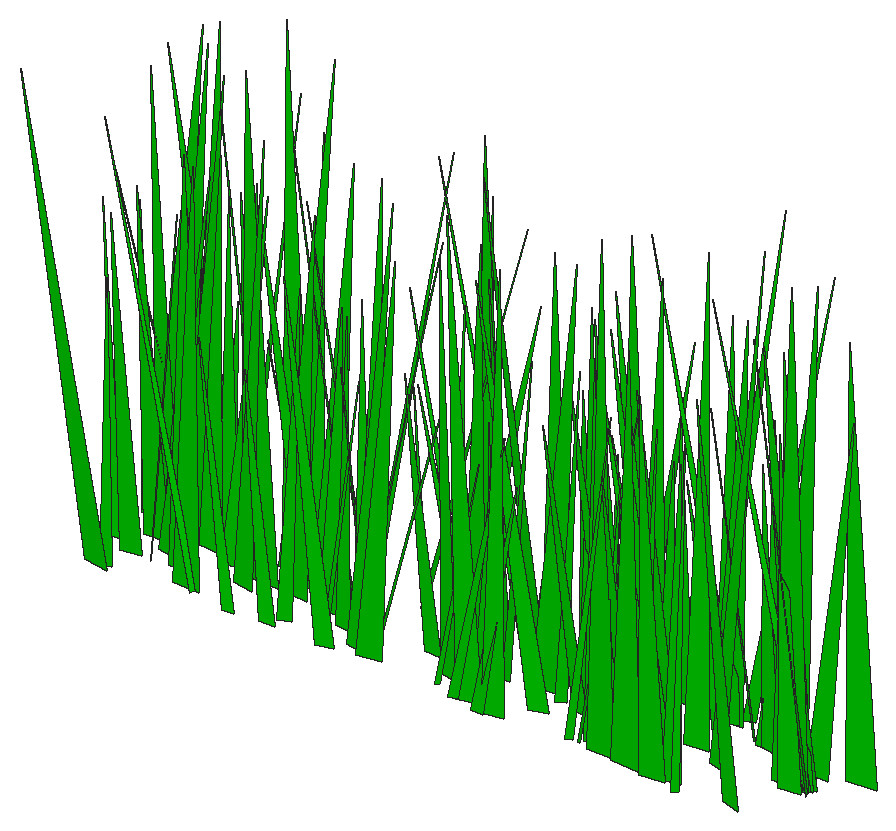
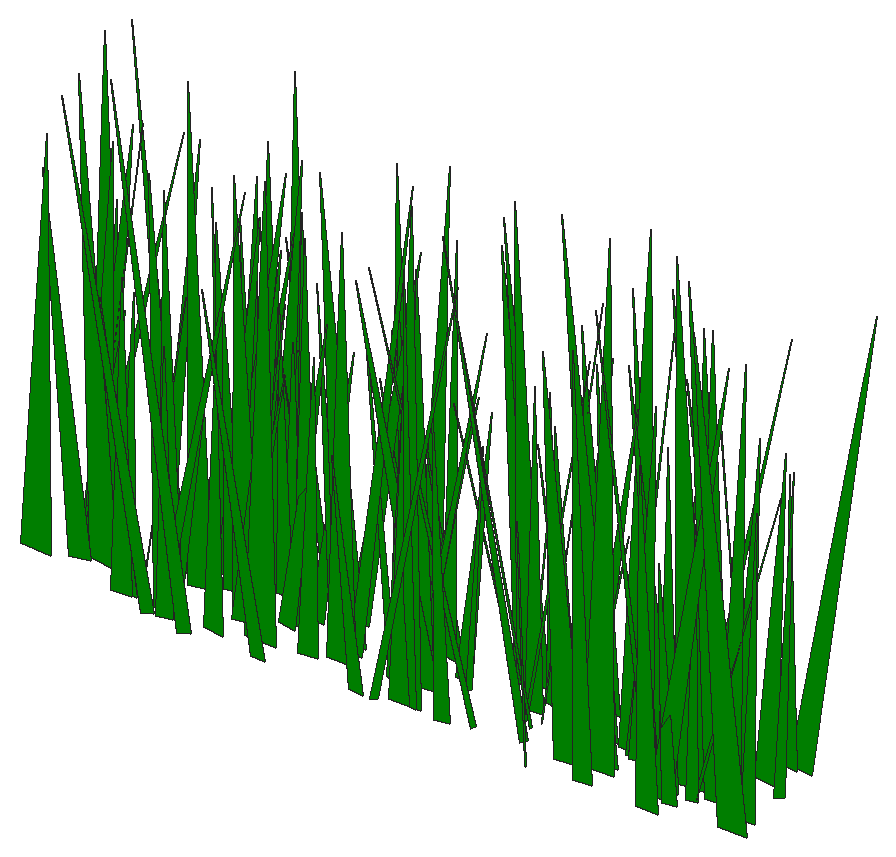
# SketchUp Ruby script. Lengths in inches.
U = 1.inch
M = Sketchup.active_model
def pt(a) = Geom::Point3d.new(a.map { |v| v * U })
def face(e, loops, mat)
  f = e.add_face(loops[0].map { |a| pt(a) })
  loops[1..].each { |l| e.add_face(l.map { |a| pt(a) }).erase! }
  f.material = f.back_material = mat if mat
  f
end
# faces: each face lists its corners as indices into pts; further lists are holes
def faces(e, pts, list, mat = nil) = list.each { |f| face(e, (f[0].is_a?(Array) ? f : [f]).map { |l| l.map { |i| pts[i] } }, mat) }
# xy, xz, yz: faces in a plane at the given z, y or x. An outline is a flat list of corners, or four numbers for a rectangle; further outlines are holes
def ring(l) = l.size == 4 ? [[l[0], l[1]], [l[2], l[1]], [l[2], l[3]], [l[0], l[3]]] : l.each_slice(2).to_a
def flat(e, list, mat, &to3) = list.each { |f| face(e, (f[0].is_a?(Array) ? f : [f]).map { |l| ring(l).map { |u, v| to3.(u, v) } }, mat) }
def xy(e, z, list, mat = nil) = flat(e, list, mat) { |x, y| [x, y, z] }
def xz(e, y, list, mat = nil) = flat(e, list, mat) { |x, z| [x, y, z] }
def yz(e, x, list, mat = nil) = flat(e, list, mat) { |y, z| [x, y, z] }
def lines(e, pts, list) = list.each { |a, b| e.add_line(pt(pts[a]), pt(pts[b])) }
# prism: a flat outline (further loops are holes) pulled along v
def prism(e, loops, v, mat = nil)
  f = face(e, loops, mat); d = Geom::Vector3d.new(v.map { |x| x * U })
  f.pushpull(f.normal.samedirection?(d) ? d.length : -d.length)
end
def box(e, o, s, mat = nil) = prism(e, [[o, [o[0] + s[0], o[1], o[2]], [o[0] + s[0], o[1] + s[1], o[2]], [o[0], o[1] + s[1], o[2]]]], [0, 0, s[2]], mat)
def at(x, y, z, deg = 0) = Geom::Transformation.translation(pt([x, y, z])) * Geom::Transformation.rotation(ORIGIN, Z_AXIS, deg.degrees)
def axes(o, x, y, z) = Geom::Transformation.new([*x, 0, *y, 0, *z, 0, *pt(o).to_a, 1])
def part(name) = M.definitions.add(name)
# library, detail: a bought-in or finely detailed component or shape, given as its bounding box
def library(name, o, s) = part(name).tap { |d| box(d.entities, o, s) }
def detail(e, o, s) = box(e.add_group.entities, o, s)
def put(e, d, t, mat = nil) = e.add_instance(d, t).tap { |i| i.material = mat if mat }
def group(e, t, mat = nil) = e.add_group.tap { |g| g.transformation = t; g.material = mat if mat }.entities
root = M.entities
M.materials.add("[Color G06]").color = [0, 204, 0]
c1 = part("fur_instance\#9")
p = [[0.8125,0,1.79],[0.67,-0.02,1.48],[0,-0.11,0],[0,0.11,0]]
faces(c1.entities,p,[[0,1,2,3]])
put(root,c1,axes([12.97,15.97,4.28],[-3.99337,-0.56787,0.77876],[-4.0854,0.55967,0.08592],[0.40602,0.04624,8.52399]),"[Color G06]")
put(root,c1,axes([12.24,19.35,4.28],[-2.73791,0.24663,2.09563],[1.98216,0.40975,0.245],[1.07946,-0.12686,4.86539]),"[Color G06]")
put(root,c1,axes([12.44,17.64,4.28],[-3.32975,0.20415,1.76228],[1.47677,0.49102,-0.30149],[1.16308,-0.03901,5.42796]),"[Color G06]")
put(root,c1,axes([14.24,19.35,4.28],[-4.0614,-0.11884,0.09777],[-0.84903,0.56603,0.25097],[0.09846,-0.02105,6.19718]),"[Color G06]")
put(root,c1,axes([12.99,19.34,4.28],[-2.92814,-0.56418,2.22224],[-4.18418,0.43225,0.29114],[1.03573,0.15122,7.45871]),"[Color G06]")
put(root,c1,axes([12.22,20.1,4.28],[2.30465,0.69491,2.08222],[5.1631,-0.32291,-0.38533],[-0.34273,-0.1917,8.19688]),"[Color G06]")
put(root,c1,axes([13.31,17.18,4.28],[-0.75917,-0.50042,1.73825],[-3.77236,0.09965,-0.38475],[-0.0241,0.16607,5.46872]),"[Color G06]")
put(root,c1,axes([13.37,18.3125,4.28],[-0.04547,-0.61844,0.06629],[-4.4314,0.00608,-0.27434],[-0.1831,0.00644,6.62305]),"[Color G06]")
put(root,c1,axes([13.24,16.09,4.28],[2.66433,-0.22899,1.74164],[-1.66367,-0.40217,-0.38923],[-1.13439,0.05198,4.66142]),"[Color G06]")
put(root,c1,axes([15.12,19.87,4.28],[-4.34443,0.46349,1.04288],[3.36999,0.60791,0.32271],[0.4215,-0.08318,8.16905]),"[Color G06]")
put(root,c1,axes([14.3,19.41,4.28],[-2.26458,0.22299,1.73631],[1.73449,0.34233,0.00285],[0.9478,-0.09368,4.14335]),"[Color G06]")
put(root,c1,axes([13.57,19.03,4.28],[3.79606,-0.59816,1.93914],[-4.37494,-0.54602,-0.21773],[-0.97142,0.12164,8.55822]),"[Color G06]")
put(root,c1,axes([16.17,16.53,4.28],[-5.20829,0.09415,0.81442],[0.69711,0.72939,0.2722],[0.51653,-0.03508,7.84458]),"[Color G06]")
put(root,c1,axes([14.06,17.17,4.28],[3.87029,0.05666,1.82111],[0.36921,-0.56575,0.26912],[-1.23022,0.00845,5.80998]),"[Color G06]")
put(root,c1,axes([14.07,17.84,4.28],[3.71321,0.3398,1.42529],[2.48378,-0.53033,0.06985],[-0.82348,-0.06738,6.63758]),"[Color G06]")
put(root,c1,axes([14.67,19.98,4.28],[1.18507,-0.32203,1.12325],[-2.4133,-0.16921,0.11452],[-0.27201,0.09828,3.87775]),"[Color G06]")
put(root,c1,axes([14.76,18.81,4.28],[-0.00288,0.78852,3.16986],[6.0329,0.01406,-0.38965],[0.27952,-0.29542,8.4424]),"[Color G06]")
put(root,c1,axes([14.98,20.64,4.28],[-0.50165,-0.47813,2.71106],[-3.86307,0.08472,0.1197],[0.35197,0.24839,5.1778]),"[Color G06]")
put(root,c1,axes([14.48,18.375,4.28],[3.8157,0.52747,2.29269],[3.94724,-0.5514,-0.10152],[-1.0396,-0.15758,8.02953]),"[Color G06]")
put(root,c1,axes([15.18,19.41,4.28],[2.12266,-0.39029,2.66699],[-3.16809,-0.32635,0.14609],[-0.99052,0.20743,5.24802]),"[Color G06]")
put(root,c1,axes([15.22,17.28,4.28],[0.01322,-0.6977,1.04536],[-5.04951,0.00129,0.24114],[0.16106,0.09754,7.47412]),"[Color G06]")
put(root,c1,axes([15.85,16.57,4.28],[1.1157,0.61922,2.23173],[4.66513,-0.1665,0.09743],[-0.43033,-0.1996,6.84238]),"[Color G06]")
put(root,c1,axes([15.36,20.01,4.28],[5.25298,-0.04802,1.83643],[-0.34875,-0.75223,-0.03124],[-1.22749,0.00822,7.86775]),"[Color G06]")
put(root,c1,axes([16.93,18.49,4.28],[-1.99698,0.53565,0.90443],[3.86216,0.28426,-0.29118],[0.45339,-0.06214,6.46403]),"[Color G06]")
put(root,c1,axes([17.51,18.43,4.28],[-5.08262,-0.02922,1.9462],[-0.14859,0.73101,0.39401],[1.31053,-0.03044,7.59258]),"[Color G06]")
put(root,c1,axes([16.02,18.39,4.28],[3.71946,-0.31875,1.53864],[-2.36483,-0.53136,0.12424],[-0.83221,0.0853,6.52372]),"[Color G06]")
put(root,c1,axes([17.72,16.2,4.28],[-2.50517,0.23981,0.70508],[1.72266,0.35476,-0.18919],[0.4611,-0.02247,4.53757]),"[Color G06]")
put(root,c1,axes([17.32,18.19,4.28],[-0.30423,-0.86212,0.93414],[-6.21332,0.04351,0.09236],[0.09275,0.08662,9.25092]),"[Color G06]")
put(root,c1,axes([17.55,19.71,4.28],[-3.56106,0.6221,3.38706],[4.81861,0.53089,0.11525],[1.34882,-0.25418,8.53056]),"[Color G06]")
put(root,c1,axes([17.12,17.66,4.28],[3.69725,0.44313,2.60223],[3.39482,-0.54489,-0.11494],[-1.26701,-0.16687,7.28555]),"[Color G06]")
put(root,c1,axes([18.66,18.76,4.28],[-3.42525,0.34148,0.96228],[2.48879,0.48185,0.14553],[0.46633,-0.06338,6.29139]),"[Color G06]")
put(root,c1,axes([17.48,20.53,4.28],[-3.57875,0.32608,3.47096],[2.71455,0.56274,0.1788],[1.86891,-0.19296,6.38681]),"[Color G06]")
put(root,c1,axes([18.64,18.99,4.28],[-2.60474,-0.11719,0.41893],[-0.83062,0.36527,0.2014],[0.30803,-0.00599,4.08561]),"[Color G06]")
put(root,c1,axes([17.59,19.36,4.28],[-3.88057,0.44362,5.32366],[3.90711,0.66294,0.01572],[2.74645,-0.31629,7.49964]),"[Color G06]")
put(root,c1,axes([19.05,16.35,4.28],[-1.44782,0.36298,0.04776],[2.60234,0.20194,-0.088],[0.06699,0.0001,4.45081]),"[Color G06]")
put(root,c1,axes([18.53,19.875,4.28],[0.32232,0.67897,0.85695],[4.8979,-0.04104,-0.3795],[0.21728,-0.08203,7.28323]),"[Color G06]")
put(root,c1,axes([18.58,18.17,4.28],[1.04511,-0.6508,0.62458],[-4.68306,-0.14307,0.37927],[0.15738,0.06455,7.13791]),"[Color G06]")
put(root,c1,axes([20.64,18.48,4.28],[-5.04728,-0.06519,1.53889],[-0.4679,0.71828,0.06742],[1.02946,0.00685,7.57553]),"[Color G06]")
put(root,c1,axes([19.39,20.82,4.28],[2.51743,0.06611,1.50259],[0.57866,-0.37429,-0.27395],[-0.94903,-0.05286,3.8188]),"[Color G06]")
put(root,c1,axes([19.35,16.8125,4.28],[3.03443,-0.31056,1.66408],[-2.27883,-0.44502,-0.25852],[-1.00338,0.07149,5.61967]),"[Color G06]")
put(root,c1,axes([21.03,18.76,4.28],[-4.51249,0.00468,1.04323],[0.02243,0.63665,-0.11127],[0.69846,0.00978,6.74352]),"[Color G06]")
put(root,c1,axes([20.08,18.02,4.28],[0.23374,0.52169,0.02925],[3.74089,-0.03263,0.07414],[-0.05073,-0.00229,5.60188]),"[Color G06]")
put(root,c1,axes([21.22,16.33,4.28],[-2.97507,0.39241,0.93894],[2.85386,0.41871,0.09665],[0.41139,-0.06682,6.11972]),"[Color G06]")
put(root,c1,axes([20.39,17.47,4.28],[2.87267,-0.04954,0.94055],[-0.36714,-0.40987,0.02501],[-0.62244,0.01314,4.32605]),"[Color G06]")
put(root,c1,axes([20.95,17.52,4.28],[2.15661,0.34791,2.0146],[2.6896,-0.32579,0.03183],[-0.89886,-0.1401,4.9288]),"[Color G06]")
put(root,c1,axes([21.24,18.13,4.28],[-2.20847,0.34506,2.4406],[2.79412,0.33718,0.17148],[0.99128,-0.18166,4.95408]),"[Color G06]")
put(root,c1,axes([21.89,17.42,4.28],[-2.90538,-0.03584,1.2201],[-0.2819,0.42045,-0.08058],[0.80811,0.01781,4.35853]),"[Color G06]")
put(root,c1,axes([20.33,19.71,4.28],[5.4871,-0.11222,1.2148],[-0.82981,-0.77282,0.17144],[-0.78721,0.03244,8.28684]),"[Color G06]")
put(root,c1,axes([20.67,18.96,4.28],[4.7064,0.0037,0.7795],[0.04286,-0.65997,-0.21778],[-0.52047,-0.02085,7.03079]),"[Color G06]")
put(root,c1,axes([22.3125,16.98,4.28],[-3.43987,0.47523,3.74009],[3.79084,0.54588,-0.17991],[1.87253,-0.2321,7.23484]),"[Color G06]")
put(root,c1,axes([22.05,16.8,4.28],[3.64569,0.49267,2.10372],[3.67873,-0.52579,-0.09533],[-0.96466,-0.14321,7.58698]),"[Color G06]")
put(root,c1,axes([22.95,20.28,4.28],[2.39811,-0.32059,1.90981],[-2.47886,-0.3561,0.08587],[-0.87967,0.12949,4.96445]),"[Color G06]")
put(root,c1,axes([23.5,18.3125,4.28],[-2.61944,0.11067,1.29609],[0.79209,0.3844,-0.19463],[0.86861,-0.01679,4.08605]),"[Color G06]")
put(root,c1,axes([22.67,16.6,4.28],[2.58776,-0.57387,1.0544],[-4.14768,-0.36661,-0.18318],[-0.48026,0.07406,7.26333]),"[Color G06]")
put(root,c1,axes([23.98,17.95,4.28],[-1.29592,-0.41524,0.6149],[-3.0044,0.181,-0.1027],[0.10063,0.05645,4.85264]),"[Color G06]")
put(root,c1,axes([22.4,17.375,4.28],[3.16952,0.08118,0.18889],[0.58245,-0.44232,0.00692],[-0.12514,-0.00255,4.81633]),"[Color G06]")
put(root,c1,axes([25.35,20.44,4.28],[-5.24058,0.10532,0.92421],[0.76645,0.73558,0.0781],[0.60452,-0.01956,7.91298]),"[Color G06]")
put(root,c1,axes([22,19.98,4.28],[5.15965,-0.04603,0.24118],[-0.3322,-0.71977,0.09534],[-0.15695,0.01032,7.72665]),"[Color G06]")
put(root,c1,axes([25.55,17.91,4.28],[-4.16168,0.10609,0.76813],[0.76342,0.58466,-0.03662],[0.50999,-0.0095,6.3229]),"[Color G06]")
put(root,c1,axes([24.23,20.17,4.28],[3.89408,0.32417,2.95544],[2.58214,-0.58824,-0.1877],[-1.62702,-0.1577,6.77562]),"[Color G06]")
put(root,c1,axes([24.41,20.16,4.28],[-1.14896,-0.74215,2.53014],[-5.56478,0.17257,0.17026],[0.47377,0.22719,8.13583]),"[Color G06]")
put(root,c1,axes([24.89,18.74,4.28],[2.16476,0.52445,2.62984],[4.06025,-0.32528,-0.01402],[-0.86901,-0.21336,6.48561]),"[Color G06]")
put(root,c1,axes([26.1,17.25,4.28],[-2.88067,0.24068,0.35111],[1.7402,0.40043,0.36019],[0.07683,-0.04569,5.00608]),"[Color G06]")
put(root,c1,axes([25.18,17.17,4.28],[3.36748,0.36101,3.26227],[2.94574,-0.52402,-0.13064],[-1.67019,-0.19634,6.34706]),"[Color G06]")
put(root,c1,axes([25.68,19.23,4.28],[-3.57116,-0.23033,2.25433],[-1.85175,0.52669,-0.37073],[1.25476,0.12174,5.86893]),"[Color G06]")
put(root,c1,axes([24.4,19.02,4.28],[3.76842,-0.38067,0.08752],[-2.7303,-0.52551,0.02879],[-0.03612,0.00697,6.95467]),"[Color G06]")
put(root,c1,axes([26.02,18.2,4.28],[-2.36297,-0.15451,1.64195],[-1.20853,0.35708,-0.02501],[0.98696,0.06733,3.90053]),"[Color G06]")
put(root,c1,axes([25.16,16.67,4.28],[2.75052,-0.07469,0.51501],[-0.53119,-0.38654,-0.10239],[-0.35132,-0.00027,4.18681]),"[Color G06]")
put(root,c1,axes([26.57,16.4,4.28],[-3.66563,0.4997,2.75267],[3.85257,0.53635,0.27512],[1.17942,-0.19892,7.65655]),"[Color G06]")
put(root,c1,axes([26,20.48,4.28],[1.29119,0.3455,0.36803],[2.48288,-0.18156,0.12241],[-0.18666,-0.02514,4.17395]),"[Color G06]")
put(root,c1,axes([27.44,18.71,4.28],[-4.81347,-0.39314,1.65522],[-2.82911,0.6871,0.36968],[1.08214,0.04763,8.32904]),"[Color G06]")
put(root,c1,axes([26.52,17.24,4.28],[1.15356,-0.50879,1.09317],[-3.71894,-0.16141,0.13585],[-0.13219,0.10111,5.71768]),"[Color G06]")
put(root,c1,axes([26.58,18.1,4.28],[3.17916,0.25116,1.41806],[1.79703,-0.46151,0.39087],[-0.9566,-0.03227,5.44706]),"[Color G06]")
put(root,c1,axes([26.05,16.3,4.28],[3.09991,-0.2022,0.39382],[-1.45116,-0.43371,-0.06535],[-0.25724,0.01003,5.11445]),"[Color G06]")
put(root,c1,axes([28.51,17.21,4.28],[-3.71731,0.43062,0.59629],[3.10304,0.5195,0.11403],[0.25793,-0.04376,7.22186]),"[Color G06]")
put(root,c1,axes([27.46,19.34,4.28],[0.04217,-0.66337,1.82671],[-4.91117,-0.00322,0.11907],[0.07142,0.17051,7.10924]),"[Color G06]")
put(root,c1,axes([27.13,16.07,4.28],[1.7386,0.32911,0.00623],[2.35863,-0.24231,0.15265],[-0.0847,0.00798,4.37852]),"[Color G06]")
put(root,c1,axes([27.62,16.17,4.28],[3.51083,-0.45343,2.81826],[-3.48747,-0.52717,-0.03872],[-1.40235,0.17582,7.15191]),"[Color G06]")
put(root,c1,axes([28.45,19.65,4.28],[-0.43724,-0.48819,0.48954],[-3.50938,0.06346,0.26863],[0.21966,0.04214,5.26624]),"[Color G06]")
put(root,c1,axes([27.9,18.34,4.28],[2.19793,-0.70483,0.35704],[-5.05855,-0.30697,-0.05166],[-0.12699,0.02862,8.23749]),"[Color G06]")
put(root,c1,axes([29.52,17.89,4.28],[-1.98109,-0.37435,0.48553],[-2.69363,0.27813,0.08393],[0.23827,0.03177,4.9858]),"[Color G06]")
put(root,c1,axes([28.68,18.0625,4.28],[3.38444,-0.21962,1.72049],[-1.60433,-0.49622,-0.22711],[-1.10991,0.04757,5.57456]),"[Color G06]")
put(root,c1,axes([30.04,18.66,4.28],[-2.17423,-0.41258,0.76693],[-2.99199,0.30516,-0.08877],[0.2555,0.06261,5.48688]),"[Color G06]")
put(root,c1,axes([29.46,18.51,4.28],[1.2325,0.57157,2.16422],[4.30418,-0.18989,0.28582],[-0.60989,-0.18507,6.39069]),"[Color G06]")
put(root,c1,axes([30.09,19.84,4.28],[-0.15315,-0.68705,2.67581],[-5.24219,0.0209,-0.05361],[0.01748,0.24969,7.36715]),"[Color G06]")
put(root,c1,axes([31.13,19.22,4.28],[-2.47487,0.59914,0.02513],[4.29363,0.34497,-0.26384],[0.16136,0.01026,7.40604]),"[Color G06]")
put(root,c1,axes([29.47,20.71,4.28],[3.1825,0.36757,0.87629],[2.67812,-0.44581,-0.24469],[-0.34571,-0.06987,6.17127]),"[Color G06]")
put(root,c1,axes([31.43,19.1,4.28],[-2.67538,0.22308,0.53204],[1.62152,0.3741,0.19492],[0.23789,-0.04116,4.65479]),"[Color G06]")
put(root,c1,axes([30.94,16.72,4.28],[3.06671,-0.33736,2.7629],[-2.72528,-0.46729,0.20242],[-1.35768,0.17597,5.83448]),"[Color G06]")
put(root,c1,axes([30.23,16.48,4.28],[3.76639,-0.13217,1.20525],[-0.96093,-0.53663,-0.05273],[-0.79079,0.02257,5.80443]),"[Color G06]")
put(root,c1,axes([31.22,17.27,4.28],[1.97021,-0.33519,1.64699],[-2.53812,-0.29348,-0.07908],[-0.74188,0.11387,4.64449]),"[Color G06]")
put(root,c1,axes([31.5,16.57,4.28],[-0.15398,0.42548,0.18327],[3.05228,0.02093,0.1467],[-0.09193,-0.01776,4.56368]),"[Color G06]")
put(root,c1,axes([31.52,20.23,4.28],[0.65567,0.43101,1.35597],[3.19532,-0.10338,0.32354],[-0.40815,-0.11695,4.71125]),"[Color G06]")
put(root,c1,axes([31.47,16.4,4.28],[3.0712,0.62728,3.17092],[4.76894,-0.47012,0.36582],[-1.41202,-0.22343,8.13241]),"[Color G06]")
put(root,c1,axes([31.38,18.82,4.28],[1.0346,0.69031,1.49059],[5.03848,-0.15064,0.20224],[-0.33896,-0.13215,7.5559]),"[Color G06]")
put(root,c1,axes([31.55,17.25,4.28],[0.61246,-0.35566,1.05629],[-2.63957,-0.08948,-0.04241],[-0.19359,0.09487,3.92012]),"[Color G06]")
put(root,c1,axes([32.17,16.46,4.28],[2.68438,-0.43992,3.9778],[-3.71413,-0.45057,-0.12542],[-1.80038,0.27358,6.18967]),"[Color G06]")
put(root,c1,axes([30.58,16.52,4.28],[4.05523,0.12048,0.92255],[0.841,-0.57188,0.32168],[-0.64825,0.01177,6.18851]),"[Color G06]")
put(root,c1,axes([32.29,17.36,4.28],[-3.02264,-0.17933,1.20075],[-1.30641,0.43482,0.11388],[0.76979,0.03378,4.90811]),"[Color G06]")
put(root,c1,axes([31.48,16.47,4.28],[2.58244,-0.19784,1.46172],[-1.53046,-0.37624,0.18993],[-0.7919,0.08197,4.39967]),"[Color G06]")
put(root,c1,axes([33.46,20.23,4.28],[-5.24909,0.19126,0.84342],[1.36531,0.73618,-0.1972],[0.57936,-0.00199,8.10616]),"[Color G06]")
put(root,c1,axes([32.34,16.59,4.28],[-1.46668,-0.43821,0.1902],[-3.13231,0.20529,0.37872],[0.28345,0.00108,5.16925]),"[Color G06]")
put(root,c1,axes([33.47,16.6,4.28],[-3.5207,0.32723,0.7119],[2.36649,0.49352,0.08366],[0.36508,-0.04337,6.32309]),"[Color G06]")
put(root,c1,axes([33.58,16.64,4.28],[-3.31135,0.51856,0.73563],[3.73861,0.46371,0.04202],[0.30622,-0.05388,7.44186]),"[Color G06]")
put(root,c1,axes([32.53,16.26,4.28],[-0.43219,-0.64999,1.96],[-4.82871,0.07157,0.34818],[0.36182,0.17875,6.98784]),"[Color G06]")
put(root,c1,axes([32.5625,18.01,4.28],[-0.50448,0.42523,1.54657],[3.19687,0.08369,-0.31414],[0.38719,-0.13699,4.60886]),"[Color G06]")
put(root,c1,axes([33.23,17.41,4.28],[-1.53064,-0.57222,0.55599],[-4.1156,0.21498,0.1081],[0.198,0.04506,6.54491]),"[Color G06]")
put(root,c1,axes([33.14,20.49,4.28],[-1.33643,0.3862,1.20362],[2.83094,0.19933,-0.32577],[0.55204,-0.08723,4.58445]),"[Color G06]")
put(root,c1,axes([33.94,19,4.28],[-1.82838,0.32675,0.41828],[2.35982,0.25351,0.29161],[0.01729,-0.04751,4.43252]),"[Color G06]")
put(root,c1,axes([33.01,16.45,4.28],[3.26554,-0.22757,2.19486],[-1.8401,-0.4839,0.35181],[-1.19749,0.123,5.44477]),"[Color G06]")
put(root,c1,axes([33.23,20.11,4.28],[2.63146,-0.52644,1.9574],[-3.87525,-0.38954,-0.39767],[-0.97461,0.12751,6.86626]),"[Color G06]")
put(root,c1,axes([33.59,16.19,4.28],[-0.38611,0.51168,3.55832],[4.37407,0.04551,0.30847],[0.00447,-0.33324,5.50577]),"[Color G06]")
put(root,c1,axes([32.13,20.85,4.28],[5.75361,-0.25016,1.67822],[-1.84183,-0.81526,0.14501],[-1.04246,0.05974,9.00631]),"[Color G06]")
put(root,c1,axes([33.45,18.43,4.28],[4.0717,-0.46944,3.21979],[-3.67205,-0.6087,0.17779],[-1.57804,0.20518,7.89407]),"[Color G06]")
put(root,c1,axes([34.52,19.79,4.28],[-3.59583,-0.03584,1.08931],[-0.31038,0.50993,-0.36157],[0.70776,0.04156,5.3758]),"[Color G06]")
put(root,c1,axes([33.22,20.17,4.28],[1.69267,-0.67903,0.33231],[-4.87284,-0.23658,-0.0885],[-0.12898,0.02657,7.70444]),"[Color G06]")
put(root,c1,axes([34.19,16.34,4.28],[-1.96569,0.34586,2.93287],[2.95239,0.31619,0.13681],[1.13394,-0.22369,4.72796]),"[Color G06]")
put(root,c1,axes([34.61,15.98,4.28],[-3.47131,0.11416,2.7309],[0.91712,0.54398,-0.00824],[1.77984,-0.05765,5.33045]),"[Color G06]")
put(root,c1,axes([35.02,20.15,4.28],[-0.92996,0.46945,1.62053],[3.51803,0.13889,-0.11249],[0.3646,-0.14278,5.21882]),"[Color G06]")
put(root,c1,axes([35.28,19.59,4.28],[-1.20549,-0.42802,1.06817],[-3.1126,0.17843,0.36657],[0.49413,0.07971,4.91502]),"[Color G06]")
put(root,c1,axes([34.84,20.0625,4.28],[1.25524,0.42183,0.77034],[3.0675,-0.17459,-0.18246],[-0.08326,-0.07294,4.89152]),"[Color G06]")
put(root,c1,axes([33.7,20.58,4.28],[5.47503,-0.22608,1.01484],[-1.63772,-0.76861,0.06657],[-0.63831,0.03288,8.53381]),"[Color G06]")
put(root,c1,axes([34.65,17.89,4.28],[5.1939,0.39681,2.3982],[2.94901,-0.75032,-0.00506],[-1.40555,-0.10794,8.85136]),"[Color G06]")
put(root,c1,axes([35.05,19.63,4.28],[1.77292,-0.37697,0.60655],[-2.73303,-0.24588,0.28985],[-0.05872,0.06218,4.82306]),"[Color G06]")
put(root,c1,axes([37.63,18.41,4.28],[-5.36777,0.1618,0.52821],[1.14969,0.74995,-0.29238],[0.38664,0.01631,8.20261]),"[Color G06]")
put(root,c1,axes([36.4,16.32,4.28],[3.01263,0.31368,4.02546],[2.90178,-0.50104,-0.36589],[-1.97338,-0.25788,5.60738]),"[Color G06]")
put(root,c1,axes([37.13,19,4.28],[-1.81974,0.36799,0.35202],[2.64941,0.25253,0.26799],[-0.01452,-0.04123,4.78344]),"[Color G06]")
put(root,c1,axes([37.33,18.54,4.28],[-1.50871,-0.66813,1.28223],[-4.86753,0.2073,-0.38491],[0.00813,0.1249,7.49775]),"[Color G06]")
put(root,c1,axes([37.73,18.23,4.28],[-4.92287,-0.0516,1.71388],[-0.3541,0.70484,0.16585],[1.15176,-0.00386,7.37649]),"[Color G06]")
put(root,c1,axes([37.24,18.4375,4.28],[-1.44017,0.66163,0.98939],[4.78713,0.20245,0.01319],[0.18375,-0.08869,7.41076]),"[Color G06]")
put(root,c1,axes([36.49,19.1,4.28],[2.35319,0.70484,1.73986],[5.14348,-0.34012,0.28902],[-0.67012,-0.13545,8.32806]),"[Color G06]")
put(root,c1,axes([37.19,18.09,4.28],[-1.69467,0.47814,1.83946],[3.60508,0.24735,0.03306],[0.52448,-0.15529,5.7163]),"[Color G06]")
put(root,c1,axes([37.03,18.33,4.28],[0.7159,-0.81809,1.49443],[-5.95062,-0.1006,0.04137],[-0.09325,0.13888,8.83323]),"[Color G06]")
put(root,c1,axes([37.28,19.25,4.28],[2.67013,-0.46839,1.20258],[-3.43692,-0.37438,0.2956],[-0.34265,0.1052,6.40627]),"[Color G06]")
put(root,c1,axes([38.62,19.66,4.28],[-0.89679,0.70548,0.77293],[5.08552,0.12415,0.16309],[-0.01775,-0.07366,7.67747]),"[Color G06]")
